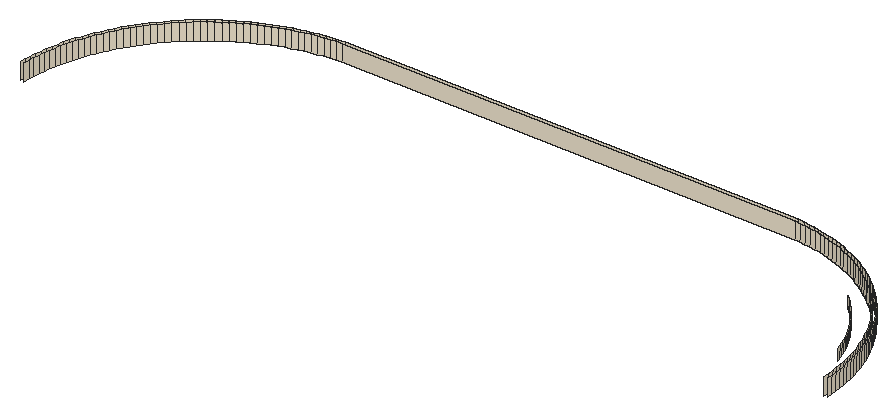
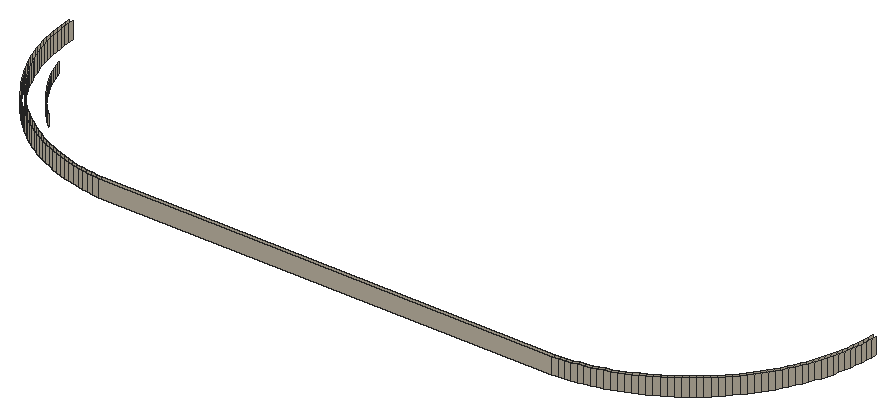
# SketchUp Ruby script. Lengths in inches.
U = 1.inch
M = Sketchup.active_model
def pt(a) = Geom::Point3d.new(a.map { |v| v * U })
def face(e, loops, mat)
  f = e.add_face(loops[0].map { |a| pt(a) })
  loops[1..].each { |l| e.add_face(l.map { |a| pt(a) }).erase! }
  f.material = f.back_material = mat if mat
  f
end
# faces: each face lists its corners as indices into pts; further lists are holes
def faces(e, pts, list, mat = nil) = list.each { |f| face(e, (f[0].is_a?(Array) ? f : [f]).map { |l| l.map { |i| pts[i] } }, mat) }
# xy, xz, yz: faces in a plane at the given z, y or x. An outline is a flat list of corners, or four numbers for a rectangle; further outlines are holes
def ring(l) = l.size == 4 ? [[l[0], l[1]], [l[2], l[1]], [l[2], l[3]], [l[0], l[3]]] : l.each_slice(2).to_a
def flat(e, list, mat, &to3) = list.each { |f| face(e, (f[0].is_a?(Array) ? f : [f]).map { |l| ring(l).map { |u, v| to3.(u, v) } }, mat) }
def xy(e, z, list, mat = nil) = flat(e, list, mat) { |x, y| [x, y, z] }
def xz(e, y, list, mat = nil) = flat(e, list, mat) { |x, z| [x, y, z] }
def yz(e, x, list, mat = nil) = flat(e, list, mat) { |y, z| [x, y, z] }
def lines(e, pts, list) = list.each { |a, b| e.add_line(pt(pts[a]), pt(pts[b])) }
# prism: a flat outline (further loops are holes) pulled along v
def prism(e, loops, v, mat = nil)
  f = face(e, loops, mat); d = Geom::Vector3d.new(v.map { |x| x * U })
  f.pushpull(f.normal.samedirection?(d) ? d.length : -d.length)
end
def box(e, o, s, mat = nil) = prism(e, [[o, [o[0] + s[0], o[1], o[2]], [o[0] + s[0], o[1] + s[1], o[2]], [o[0], o[1] + s[1], o[2]]]], [0, 0, s[2]], mat)
def at(x, y, z, deg = 0) = Geom::Transformation.translation(pt([x, y, z])) * Geom::Transformation.rotation(ORIGIN, Z_AXIS, deg.degrees)
def axes(o, x, y, z) = Geom::Transformation.new([*x, 0, *y, 0, *z, 0, *pt(o).to_a, 1])
def part(name) = M.definitions.add(name)
# library, detail: a bought-in or finely detailed component or shape, given as its bounding box
def library(name, o, s) = part(name).tap { |d| box(d.entities, o, s) }
def detail(e, o, s) = box(e.add_group.entities, o, s)
def put(e, d, t, mat = nil) = e.add_instance(d, t).tap { |i| i.material = mat if mat }
def group(e, t, mat = nil) = e.add_group.tap { |g| g.transformation = t; g.material = mat if mat }.entities
root = M.entities
M.materials.add("0961 AP 7892 PALE IVORY").color = [243, 232, 209]
xz(root,162.63,[[76.0625,113.78,158.15,116.78]],"0961 AP 7892 PALE IVORY")
xz(root,163.26,[[76.04,113.78,158.18,116.78]],"0961 AP 7892 PALE IVORY")
p = [[43.8,131.07,113.78],[43.76,130.04,113.78],[43.76,130.04,116.78],[43.8,131.07,116.78],[44.39,130.02,113.78],[44.43,131.03,113.78],
  [44.43,131.03,116.78],[44.39,130.02,116.78],[189.57,131.02,113.78],[189.62,130.01,113.78],[189.62,130.01,116.78],[189.57,131.02,116.78],
  [190.24,130.03,113.78],[190.2,131.0625,113.78],[190.2,131.0625,116.78],[190.24,130.03,116.78],[44.51,132.05,113.78],[44.51,132.05,116.78],
  [189.49,132.03,113.78],[189.49,132.03,116.78],[43.88,132.1,113.78],[43.88,132.1,116.78],[190.12,132.09,113.78],[190.12,132.09,116.78],
  [44.62,133.06,113.78],[44.62,133.06,116.78],[189.39,133.04,113.78],[189.39,133.04,116.78],[43.99,133.13,113.78],[43.99,133.13,116.78],
  [190.01,133.11,113.78],[190.01,133.11,116.78],[189.25,134.04,113.78],[189.25,134.04,116.78],[44.13,134.16,113.78],[44.13,134.16,116.78],
  [44.75,134.0625,113.78],[44.75,134.0625,116.78],[189.875,134.14,113.78],[189.875,134.14,116.78],[189.08,135.04,113.78],[189.08,135.04,116.78],
  [44.92,135.07,113.78],[44.92,135.07,116.78],[189.7,135.15,113.78],[189.7,135.15,116.78],[44.3,135.18,113.78],[44.3,135.18,116.78],
  [188.89,136.03,113.78],[188.89,136.03,116.78],[45.12,136.0625,113.78],[45.12,136.0625,116.78],[44.5,136.2,113.78],[44.5,136.2,116.78],
  [189.5,136.17,113.78],[189.5,136.17,116.78],[188.66,137.02,113.78],[188.66,137.02,116.78],[45.35,137.05,113.78],[45.35,137.05,116.78],
  [44.74,137.21,113.78],[44.74,137.21,116.78],[189.27,137.17,113.78],[189.27,137.17,116.78],[188.41,138,113.78],[188.41,138,116.78],
  [45.61,138.04,113.78],[45.61,138.04,116.78],[45,138.21,113.78],[45,138.21,116.78],[189.01,138.17,113.78],[189.01,138.17,116.78],
  [45.89,139.01,113.78],[45.89,139.01,116.78],[188.12,138.97,113.78],[188.12,138.97,116.78],[45.29,139.2,113.78],[45.29,139.2,116.78],
  [188.72,139.16,113.78],[188.72,139.16,116.78],[46.21,139.98,113.78],[46.21,139.98,116.78],[184.97,138.96,113.78],[184.66,139.83,113.78],
  [184.66,139.83,115.78],[184.97,138.96,115.78],[187.81,139.93,113.78],[187.81,139.93,116.78],[45.61,140.18,113.78],[45.61,140.18,116.78],
  [188.4,140.14,113.78],[188.4,140.14,116.78],[184.32,140.6875,113.78],[184.32,140.6875,115.78],[187.46,140.89,113.78],[187.46,140.89,116.78],
  [46.56,140.93,113.78],[46.56,140.93,116.78],[188.05,141.11,113.78],[188.05,141.11,116.78],[45.97,141.16,113.78],[45.97,141.16,116.78],
  [183.96,141.53,113.78],[183.96,141.53,115.78],[46.93,141.88,113.78],[46.93,141.88,116.78],[187.09,141.83,113.78],[187.09,141.83,116.78],
  [187.68,142.07,113.78],[187.68,142.07,116.78],[46.35,142.12,113.78],[46.35,142.12,116.78],[183.57,142.37,113.78],[183.57,142.37,115.78],
  [186.69,142.76,113.78],[186.69,142.76,116.78],[47.33,142.8125,113.78],[47.33,142.8125,116.78],[46.76,143.07,113.78],[46.76,143.07,116.78],
  [187.27,143.02,113.78],[187.27,143.02,116.78],[183.15,143.19,113.78],[183.15,143.19,115.78],[47.76,143.73,113.78],[47.76,143.73,116.78],
  [186.27,143.68,113.78],[186.27,143.68,116.78],[186.83,143.95,113.78],[186.83,143.95,116.78],[47.2,144.01,113.78],[47.2,144.01,116.78],
  [182.71,144,113.78],[182.71,144,115.78],[48.22,144.64,113.78],[48.22,144.64,116.78],[185.8125,144.58,113.78],[185.8125,144.58,116.78],
  [47.66,144.93,113.78],[47.66,144.93,116.78],[182.25,144.8,113.78],[182.25,144.8,115.78],[186.37,144.87,113.78],[186.37,144.87,116.78],
  [48.71,145.53,113.78],[48.71,145.53,116.78],[185.33,145.47,113.78],[185.33,145.47,116.78],[181.76,145.59,113.78],[181.76,145.59,115.78],
  [48.16,145.84,113.78],[48.16,145.84,116.78],[185.88,145.78,113.78],[185.88,145.78,116.78],[49.22,146.41,113.78],[49.22,146.41,116.78],
  [184.82,146.35,113.78],[184.82,146.35,116.78],[181.25,146.35,113.78],[181.25,146.35,115.78],[48.68,146.74,113.78],[48.68,146.74,116.78],
  [185.36,146.67,113.78],[185.36,146.67,116.78],[184.29,147.21,113.78],[184.29,147.21,116.78],[49.76,147.28,113.78],[49.76,147.28,116.78],
  [180.72,147.11,113.78],[180.72,147.11,115.78],[49.23,147.62,113.78],[49.23,147.62,116.78],[184.82,147.55,113.78],[184.82,147.55,116.78],
  [180.17,147.84,113.78],[180.17,147.84,115.78],[183.73,148.05,113.78],[183.73,148.05,116.78],[50.32,148.12,113.78],[50.32,148.12,116.78],
  [184.25,148.41,113.78],[184.25,148.41,116.78],[49.8,148.48,113.78],[49.8,148.48,116.78],[179.59,148.5625,113.78],[179.59,148.5625,115.78],
  [50.91,148.95,113.78],[50.91,148.95,116.78],[183.15,148.875,113.78],[183.15,148.875,116.78],[183.65,149.25,113.78],[183.65,149.25,116.78],
  [50.41,149.32,113.78],[50.41,149.32,116.78],[178.99,149.26,113.78],[178.99,149.26,115.78],[51.53,149.76,113.78],[51.53,149.76,116.78],
  [182.54,149.68,113.78],[182.54,149.68,116.78],[183.03,150.07,113.78],[183.03,150.07,116.78],[51.03,150.15,113.78],[51.03,150.15,116.78],
  [178.375,149.95,113.78],[178.375,149.95,115.78],[181.9,150.47,113.78],[181.9,150.47,116.78],[52.17,150.55,113.78],[52.17,150.55,116.78],
  [177.73,150.61,113.78],[177.73,150.61,115.78],[51.68,150.95,113.78],[51.68,150.95,116.78],[182.39,150.875,113.78],[182.39,150.875,116.78],
  [181.25,151.25,113.78],[181.25,151.25,116.78],[52.83,151.32,113.78],[52.83,151.32,116.78],[177.07,151.26,113.78],[177.07,151.26,115.78],
  [181.72,151.66,113.78],[181.72,151.66,116.78],[52.36,151.74,113.78],[52.36,151.74,116.78],[180.57,152,113.78],[180.57,152,116.78],
  [53.51,152.07,113.78],[53.51,152.07,116.78],[176.4,151.88,113.78],[176.4,151.88,115.78],[53.05,152.5,113.78],[53.05,152.5,116.78],
  [181.03,152.43,113.78],[181.03,152.43,116.78],[179.86,152.72,113.78],[179.86,152.72,116.78],[54.22,152.8,113.78],[54.22,152.8,116.78],
  [180.3125,153.17,113.78],[180.3125,153.17,116.78],[53.77,153.25,113.78],[53.77,153.25,116.78],[179.14,153.43,113.78],[179.14,153.43,116.78],
  [54.95,153.51,113.78],[54.95,153.51,116.78],[54.52,153.97,113.78],[54.52,153.97,116.78],[179.58,153.89,113.78],[179.58,153.89,116.78],
  [178.4,154.12,113.78],[178.4,154.12,116.78],[55.7,154.2,113.78],[55.7,154.2,116.78],[178.82,154.59,113.78],[178.82,154.59,116.78],
  [55.28,154.67,113.78],[55.28,154.67,116.78],[177.63,154.78,113.78],[177.63,154.78,116.78],[56.47,154.86,113.78],[56.47,154.86,116.78],
  [178.04,155.26,113.78],[178.04,155.26,116.78],[56.07,155.34,113.78],[56.07,155.34,116.78],[176.85,155.42,113.78],[176.85,155.42,116.78],
  [57.26,155.5,113.78],[57.26,155.5,116.78],[56.87,156,113.78],[56.87,156,116.78],[177.24,155.92,113.78],[177.24,155.92,116.78],
  [176.05,156.04,113.78],[176.05,156.04,116.78],[58.07,156.12,113.78],[58.07,156.12,116.78],[176.42,156.54,113.78],[176.42,156.54,116.78],
  [57.7,156.62,113.78],[57.7,156.62,116.78],[175.22,156.63,113.78],[175.22,156.63,116.78],[58.9,156.71,113.78],[58.9,156.71,116.78],
  [175.59,157.15,113.78],[175.59,157.15,116.78],[58.54,157.22,113.78],[58.54,157.22,116.78],[174.39,157.2,113.78],[174.39,157.2,116.78],
  [59.74,157.27,113.78],[59.74,157.27,116.78],[174.73,157.73,113.78],[174.73,157.73,116.78],[59.4,157.8,113.78],[59.4,157.8,116.78],
  [173.53,157.74,113.78],[173.53,157.74,116.78],[60.6,157.8125,113.78],[60.6,157.8125,116.78],[172.66,158.26,113.78],[172.66,158.26,116.78],
  [173.86,158.28,113.78],[173.86,158.28,116.78],[60.28,158.35,113.78],[60.28,158.35,116.78],[61.48,158.33,113.78],[61.48,158.33,116.78],
  [62.37,158.8125,113.78],[62.37,158.8125,116.78],[171.77,158.74,113.78],[171.77,158.74,116.78],[172.97,158.8,113.78],[172.97,158.8,116.78],
  [61.17,158.875,113.78],[61.17,158.875,116.78],[170.87,159.21,113.78],[170.87,159.21,116.78],[63.28,159.27,113.78],[63.28,159.27,116.78],
  [172.07,159.3,113.78],[172.07,159.3,116.78],[62.08,159.37,113.78],[62.08,159.37,116.78],[169.96,159.64,113.78],[169.96,159.64,116.78],
  [64.2,159.7,113.78],[64.2,159.7,116.78],[171.15,159.77,113.78],[171.15,159.77,116.78],[63,159.84,113.78],[63,159.84,116.78],
  [169.03,160.05,113.78],[169.03,160.05,116.78],[65.13,160.11,113.78],[65.13,160.11,116.78],[63.94,160.28,113.78],[63.94,160.28,116.78],
  [170.22,160.22,113.78],[170.22,160.22,116.78],[168.09,160.43,113.78],[168.09,160.43,116.78],[66.08,160.48,113.78],[66.08,160.48,116.78],
  [169.28,160.63,113.78],[169.28,160.63,116.78],[64.89,160.69,113.78],[64.89,160.69,116.78],[167.14,160.78,113.78],[167.14,160.78,116.78],
  [67.03,160.83,113.78],[67.03,160.83,116.78],[168.32,161.02,113.78],[168.32,161.02,116.78],[65.85,161.07,113.78],[65.85,161.07,116.78],
  [68,161.15,113.78],[68,161.15,116.78],[166.19,161.1,113.78],[166.19,161.1,116.78],[167.35,161.375,113.78],[167.35,161.375,116.78],
  [66.83,161.43,113.78],[66.83,161.43,116.78],[165.22,161.4,113.78],[165.22,161.4,116.78],[68.97,161.4375,113.78],[68.97,161.4375,116.78],
  [67.81,161.75,113.78],[67.81,161.75,116.78],[69.95,161.7,113.78],[69.95,161.7,116.78],[164.24,161.66,113.78],[164.24,161.66,116.78],
  [166.375,161.7,113.78],[166.375,161.7,116.78],[70.95,161.93,113.78],[70.95,161.93,116.78],[163.25,161.9,113.78],[163.25,161.9,116.78],
  [165.39,162,113.78],[165.39,162,116.78],[68.8,162.05,113.78],[68.8,162.05,116.78],[71.94,162.13,113.78],[71.94,162.13,116.78],
  [162.26,162.1,113.78],[162.26,162.1,116.78],[69.8,162.31,113.78],[69.8,162.31,116.78],[164.39,162.27,113.78],[164.39,162.27,116.78],
  [72.94,162.3,113.78],[72.94,162.3,116.78],[161.27,162.28,113.78],[161.27,162.28,116.78],[70.8125,162.54,113.78],[70.8125,162.54,116.78],
  [73.95,162.4375,113.78],[73.95,162.4375,116.78],[160.26,162.42,113.78],[160.26,162.42,116.78],[163.39,162.51,113.78],[163.39,162.51,116.78],
  [74.96,162.55,113.78],[74.96,162.55,116.78],[159.26,162.54,113.78],[159.26,162.54,116.78],[71.83,162.75,113.78],[71.83,162.75,116.78],
  [76.0625,162.63,113.78],[76.0625,162.63,116.78],[158.15,162.63,113.78],[158.15,162.63,116.78],[162.38,162.72,113.78],[162.38,162.72,116.78],
  [72.85,162.92,113.78],[72.85,162.92,116.78],[161.37,162.9,113.78],[161.37,162.9,116.78],[73.875,163.0625,113.78],[73.875,163.0625,116.78],
  [160.35,163.05,113.78],[160.35,163.05,116.78],[159.32,163.16,113.78],[159.32,163.16,116.78],[74.9,163.17,113.78],[74.9,163.17,116.78],
  [76.04,163.26,113.78],[76.04,163.26,116.78],[158.18,163.26,113.78],[158.18,163.26,116.78]]
faces(root,p,[[0,1,2,3],[4,5,6,7],[8,9,10,11],[12,13,14,15],[5,16,17,6],[18,8,11,19],[20,0,3,21],[13,22,23,14],
  [16,24,25,17],[26,18,19,27],[28,20,21,29],[22,30,31,23],[32,26,27,33],[34,28,29,35],[24,36,37,25],[30,38,39,31],
  [40,32,33,41],[36,42,43,37],[38,44,45,39],[46,34,35,47],[48,40,41,49],[42,50,51,43],[52,46,47,53],[44,54,55,45],
  [56,48,49,57],[50,58,59,51],[60,52,53,61],[54,62,63,55],[64,56,57,65],[58,66,67,59],[68,60,61,69],[62,70,71,63],
  [66,72,73,67],[74,64,65,75],[76,68,69,77],[70,78,79,71],[72,80,81,73],[82,83,84,85],[86,74,75,87],[88,76,77,89],
  [78,90,91,79],[83,92,93,84],[94,86,87,95],[80,96,97,81],[90,98,99,91],[100,88,89,101],[92,102,103,93],[96,104,105,97],
  [106,94,95,107],[98,108,109,99],[110,100,101,111],[102,112,113,103],[114,106,107,115],[104,116,117,105],[118,110,111,119],[108,120,121,109],
  [112,122,123,113],[116,124,125,117],[126,114,115,127],[120,128,129,121],[130,118,119,131],[122,132,133,123],[124,134,135,125],[136,126,127,137],
  [138,130,131,139],[132,140,141,133],[128,142,143,129],[134,144,145,135],[146,136,137,147],[140,148,149,141],[150,138,139,151],[142,152,153,143],
  [144,154,155,145],[156,146,147,157],[148,158,159,149],[160,150,151,161],[152,162,163,153],[164,156,157,165],[154,166,167,155],[158,168,169,159],
  [170,160,161,171],[162,172,173,163],[168,174,175,169],[176,164,165,177],[166,178,179,167],[172,180,181,173],[182,170,171,183],[174,184,185,175],
  [178,186,187,179],[188,176,177,189],[180,190,191,181],[192,182,183,193],[184,194,195,185],[186,196,197,187],[198,188,189,199],[190,200,201,191],
  [202,192,193,203],[194,204,205,195],[206,198,199,207],[196,208,209,197],[204,210,211,205],[212,202,203,213],[200,214,215,201],[216,206,207,217],
  [208,218,219,209],[210,220,221,211],[214,222,223,215],[224,212,213,225],[226,216,217,227],[218,228,229,219],[220,230,231,221],[232,224,225,233],
  [222,234,235,223],[236,226,227,237],[228,238,239,229],[234,240,241,235],[242,232,233,243],[244,236,237,245],[238,246,247,239],[248,242,243,249],
  [240,250,251,241],[252,244,245,253],[246,254,255,247],[250,256,257,251],[258,248,249,259],[260,252,253,261],[254,262,263,255],[256,264,265,257],
  [266,258,259,267],[268,260,261,269],[262,270,271,263],[272,266,267,273],[264,274,275,265],[276,268,269,277],[270,278,279,271],[274,280,281,275],
  [282,272,273,283],[284,276,277,285],[278,286,287,279],[280,288,289,281],[290,282,283,291],[292,284,285,293],[286,294,295,287],[288,296,297,289],
  [298,290,291,299],[300,292,293,301],[294,302,303,295],[304,300,301,305],[296,306,307,297],[308,298,299,309],[302,310,311,303],[310,312,313,311],
  [314,304,305,315],[306,316,317,307],[318,308,309,319],[320,314,315,321],[312,322,323,313],[316,324,325,317],[326,318,319,327],[328,320,321,329],
  [322,330,331,323],[324,332,333,325],[334,326,327,335],[336,328,329,337],[330,338,339,331],[340,334,335,341],[332,342,343,333],[344,336,337,345],
  [338,346,347,339],[342,348,349,343],[350,340,341,351],[352,344,345,353],[346,354,355,347],[348,356,357,349],[358,350,351,359],[354,360,361,355],
  [362,352,353,363],[356,364,365,357],[366,358,359,367],[368,362,363,369],[360,370,371,361],[372,366,367,373],[370,374,375,371],[376,368,369,377],
  [364,378,379,365],[374,380,381,375],[382,376,377,383],[378,384,385,379],[386,372,373,387],[380,388,389,381],[390,382,383,391],[392,386,387,393],
  [384,394,395,385],[388,396,397,389],[398,390,391,399],[400,392,393,401],[396,402,403,397],[404,398,399,405],[394,406,407,395],[402,408,409,403],
  [410,404,405,411],[412,400,401,413],[408,414,415,409],[416,410,411,417],[406,418,419,407],[420,412,413,421],[418,422,423,419],[424,420,421,425],
  [422,426,427,423],[426,428,429,427],[430,424,425,431],[432,430,431,433],[428,434,435,429]],"0961 AP 7892 PALE IVORY")
